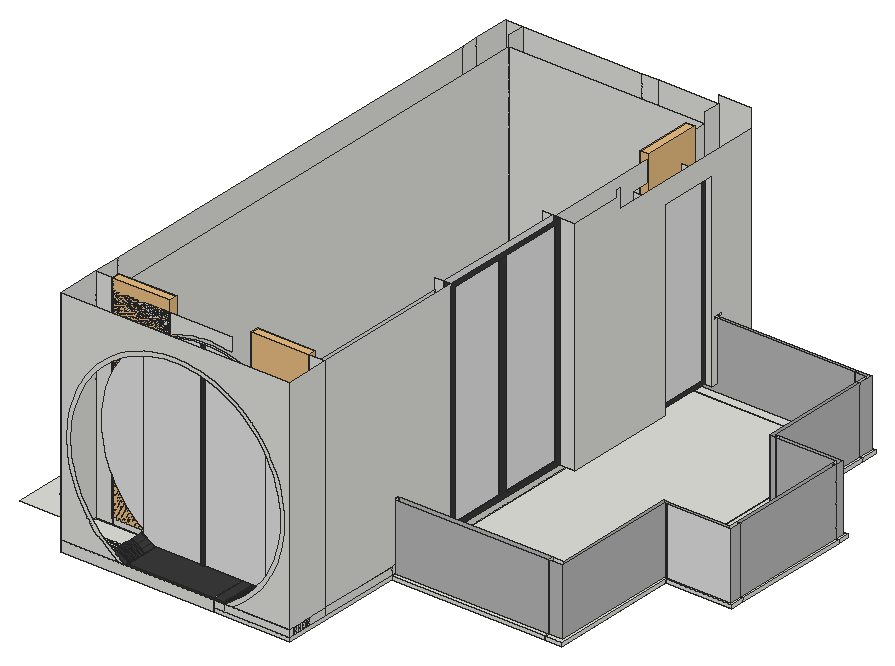
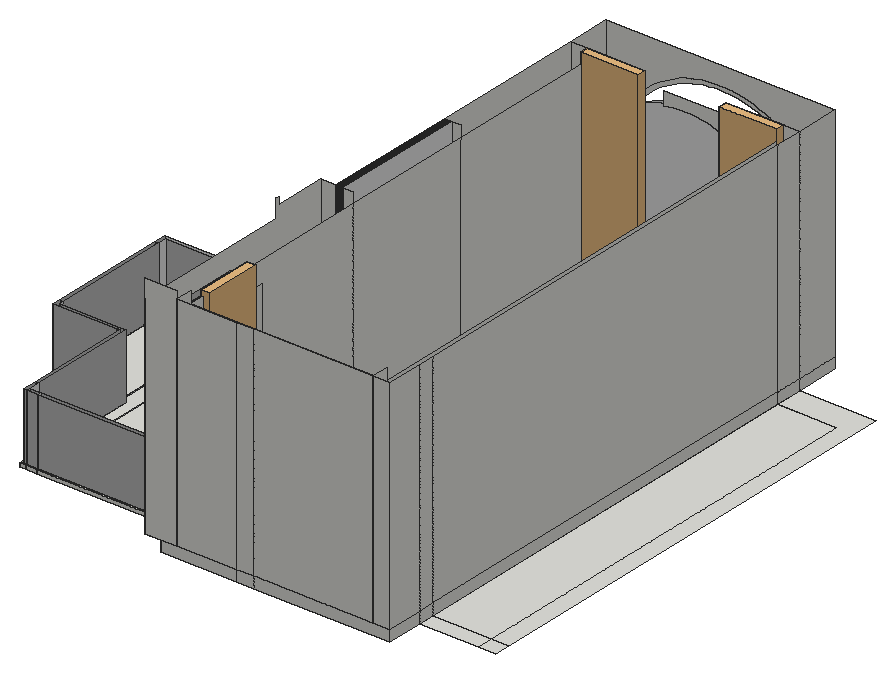
# SketchUp Ruby script. Lengths in inches.
U = 1.inch
M = Sketchup.active_model
def pt(a) = Geom::Point3d.new(a.map { |v| v * U })
def face(e, loops, mat)
  f = e.add_face(loops[0].map { |a| pt(a) })
  loops[1..].each { |l| e.add_face(l.map { |a| pt(a) }).erase! }
  f.material = f.back_material = mat if mat
  f
end
# faces: each face lists its corners as indices into pts; further lists are holes
def faces(e, pts, list, mat = nil) = list.each { |f| face(e, (f[0].is_a?(Array) ? f : [f]).map { |l| l.map { |i| pts[i] } }, mat) }
# xy, xz, yz: faces in a plane at the given z, y or x. An outline is a flat list of corners, or four numbers for a rectangle; further outlines are holes
def ring(l) = l.size == 4 ? [[l[0], l[1]], [l[2], l[1]], [l[2], l[3]], [l[0], l[3]]] : l.each_slice(2).to_a
def flat(e, list, mat, &to3) = list.each { |f| face(e, (f[0].is_a?(Array) ? f : [f]).map { |l| ring(l).map { |u, v| to3.(u, v) } }, mat) }
def xy(e, z, list, mat = nil) = flat(e, list, mat) { |x, y| [x, y, z] }
def xz(e, y, list, mat = nil) = flat(e, list, mat) { |x, z| [x, y, z] }
def yz(e, x, list, mat = nil) = flat(e, list, mat) { |y, z| [x, y, z] }
def lines(e, pts, list) = list.each { |a, b| e.add_line(pt(pts[a]), pt(pts[b])) }
# prism: a flat outline (further loops are holes) pulled along v
def prism(e, loops, v, mat = nil)
  f = face(e, loops, mat); d = Geom::Vector3d.new(v.map { |x| x * U })
  f.pushpull(f.normal.samedirection?(d) ? d.length : -d.length)
end
def box(e, o, s, mat = nil) = prism(e, [[o, [o[0] + s[0], o[1], o[2]], [o[0] + s[0], o[1] + s[1], o[2]], [o[0], o[1] + s[1], o[2]]]], [0, 0, s[2]], mat)
def at(x, y, z, deg = 0) = Geom::Transformation.translation(pt([x, y, z])) * Geom::Transformation.rotation(ORIGIN, Z_AXIS, deg.degrees)
def axes(o, x, y, z) = Geom::Transformation.new([*x, 0, *y, 0, *z, 0, *pt(o).to_a, 1])
def part(name) = M.definitions.add(name)
# library, detail: a bought-in or finely detailed component or shape, given as its bounding box
def library(name, o, s) = part(name).tap { |d| box(d.entities, o, s) }
def detail(e, o, s) = box(e.add_group.entities, o, s)
def put(e, d, t, mat = nil) = e.add_instance(d, t).tap { |i| i.material = mat if mat }
def group(e, t, mat = nil) = e.add_group.tap { |g| g.transformation = t; g.material = mat if mat }.entities
root = M.entities
M.materials.add("[Color M07]").color = [58, 58, 58]
M.materials.add("[Mirror 01]").color = [185, 185, 185]
M.materials.add("[Mirror 02]").color = [229, 229, 229]
c1 = library("Curtains 004",[-15.59,-2.26,0],[31.18,4.52,116.91])
xy(root,120,[[115,13.45,115,52.07,41.2,52.07,41.2,37.13,124,37.13,124,13.45],[41.2,13.45,115,37.13],[[115,13.45,115,37.13,41.2,37.13,41.2,295.13,115,295.13,115,315.2,124,315.2,124,295.13,165.63,295.13,165.63,106.13,126,106.13,126,82.13,165.63,82.13,165.63,13.45],[115,286.13,124,295.13]],[124,13.45,165.63,13.45,165.63,295.13,124,295.13,124,286.13,249,286.13,249,106.13,124,106.13],[0,37.13,41.2,37.13,41.2,52.07,9,52.07,9,286.13,0,286.13],
  [41.2,37.13,41.2,295.13,115,295.13,115,286.13,9,286.13,9,52.07,115,52.07,115,37.13],[126,82.13,165.63,94.13],[165.63,82.13,249,94.13],[249,82.13,258,286.13],[126,94.13,165.63,95.7],
  [165.63,94.13,249,95.7],[126,95.7,165.63,106.13],[165.63,95.7,249,106.13],[258,152.76,294,160.01],[258,160.01,294,224.82],
  [258,224.82,294,230.88],[0,286.13,9,295.13],[9,286.13,41.2,295.13],[41.2,286.13,115,295.13],[115,286.13,124,295.13],
  [124,286.13,165.63,295.13],[165.63,286.13,249,295.13],[249,286.13,255,295.13],[255,286.13,258,295.13],[115,295.13,124,315.2],
  [124,295.13,165.63,315.2]])
xy(root,122,[[124,13.45,165.63,106.13],[165.63,82.13,249,84.55],[249,82.13,258,82.13,258,153.49,256.57,153.49,256.57,84.55,249,84.55],[165.63,84.55,249,87.25],[249,84.55,249,87.25,255,87.25,255,155.13,258,155.13,258,153.49,256.57,153.49,256.57,84.55],
  [165.63,87.25,249,94.13],[249,87.25,249,286.13,255,286.13,255,227.13,258,227.13,258,155.13,255,155.13,255,87.25],[165.63,94.13,249,94.2],[165.63,94.2,238.38,95.7],[238.38,94.2,249,95.7],
  [165.63,95.7,238.38,106.13],[238.38,95.7,249,106.13],[165.63,106.13,165.63,295.13,124,295.13,124,286.13,249,286.13,249,106.13],[258,152.76,294,152.76,294,160.01,292.7,160.01,292.7,153.49,258,153.49],[258,153.49,258,155.13,290.75,155.13,290.75,160.01,292.7,160.01,292.7,153.49],
  [258,155.13,290.75,160.01],[258,160.01,290.75,224.82],[290.75,160.01,292.7,224.82],[292.7,160.01,294,224.82],[258,224.82,290.75,227.13],
  [290.75,224.82,290.75,227.13,258,227.13,258,229.11,292.7,229.11,292.7,224.82],[292.7,224.82,294,224.82,294,230.88,258,230.88,258,229.11,292.7,229.11],[255,227.13,255,286.13,256.57,286.13,256.57,229.11,258,229.11,258,227.13],[256.57,229.11,258,286.13],[165.63,286.13,249,292.13],
  [249,286.13,255,292.13],[255,286.13,256.57,293.99],[256.57,286.13,258,286.13,258,295.13,255,295.13,255,293.99,256.57,293.99],[165.63,292.13,249,293.99],[249,292.13,255,293.99],
  [165.63,293.99,249,295.13],[249,293.99,255,295.13]])
xy(root,122.625,[[165.63,87.25,249,94.13],[249,87.25,255,87.25,255,155.13,258,155.13,258,227.13,255,227.13,255,286.13,249,286.13],[165.63,94.2,238.38,95.7],[238.38,94.2,249,95.7],[165.63,95.7,238.38,106.13],
  [238.38,95.7,249,106.13],[165.63,106.13,249,106.13,249,286.13,124,286.13,124,295.13,165.63,295.13],[258,160.01,290.75,224.82]])
xy(root,126,[[41.2,13.45,77.2,14.95],[77.2,13.45,77.2,33.16,101.89,33.16,101.89,32.53,103.41,32.53,103.41,33.16,124,33.16,124,13.45],[124,13.45,129.63,33.16],[129.63,13.45,165.63,14.95],[41.2,14.95,77.2,15.8],
  [129.63,14.95,165.63,15.8],[41.2,15.8,77.2,16.65],[129.63,15.8,165.63,16.65],[41.2,16.65,77.2,17.5],[129.63,16.65,165.63,17.5],
  [41.2,17.5,77.2,18.35],[129.63,17.5,165.63,18.35],[41.2,18.35,77.2,19.21],[129.63,18.35,165.63,19.21],[41.2,19.21,77.2,19.95],
  [129.63,19.21,165.63,19.95],[41.2,19.95,77.2,21.02],[129.63,19.95,165.63,21.02],[41.2,21.02,77.2,22.08],[129.63,21.02,165.63,22.08],
  [41.2,22.08,77.2,23.14],[129.63,22.08,165.63,23.14],[41.2,23.14,77.2,24.2],[129.63,23.14,165.63,24.2],[41.2,24.2,77.2,25.27],
  [129.63,24.2,165.63,25.27],[41.2,25.27,77.2,26.33],[129.63,25.27,165.63,26.33],[41.2,26.33,77.2,37.13],[129.63,26.33,165.63,37.13],
  [101.89,32.53,103.41,33.16],[77.2,33.16,124,34.78],[124,33.16,129.63,34.78],[77.2,34.78,124,37.13],[124,34.78,129.63,37.13],
  [41.2,37.13,124,37.13,124,106.13,156.63,106.13,156.63,286.13,124,286.13,124,295.13,156.63,295.13,156.63,306.2,50.2,306.2,50.2,37.45,41.2,37.45],[124,37.13,156.63,106.13],[156.63,37.13,165.63,106.13],[41.2,37.45,50.2,315.2],[156.63,106.13,165.63,122.64],
  [156.63,122.64,161.76,196.13],[156.63,196.13,165.63,256.99],[165.63,196.13,174.13,256.99],[156.63,256.99,165.63,286.13],[124,286.13,156.63,295.13],
  [156.63,286.13,165.63,288.98],[156.63,288.98,165.63,295.13],[165.63,288.98,174.13,292.13],[165.63,293.99,174.13,295.13],[156.63,295.13,165.63,315.2],
  [165.63,295.13,174.13,315.2],[50.2,306.2,156.63,315.2]])
xy(root,126,[[161.76,122.64,165.63,196.13],[168.07,256.99,169.88,286.13],[168.07,286.13,169.88,288.98]],"[Color M07]")
xy(root,126.625,[[77.2,13.45,124,13.45,124,33.16,103.41,33.16,103.41,32.53,101.89,32.53,101.89,33.16,77.2,33.16],[124,13.45,129.63,33.16]],"[Color M07]")
xy(root,127.86,[[169.38,258.85,169.88,286.13],[169.38,286.13,169.88,287.12]],"[Color M07]")
xy(root,128.57,[[164.38,125.2,165.63,155.73],[164.38,159.39,165.63,193.57]],"[Color M07]")
xz(root,13.45,[[41.2,120,124,126],[124,120,165.63,122],[124,122,129.63,126],[129.63,122,165.63,126],[41.2,126,72.37,126,69.11,128.28,68.1,128.99,65.61,130.93,63.22,133.01,60.95,135.22,58.8,137.54,56.78,139.97,54.89,142.51,53.13,145.14,51.52,147.86,50.06,150.67,48.75,153.55,47.59,156.49,46.59,159.49,45.75,162.54,45.08,165.64,44.57,168.76,44.23,171.9,44.0625,175.0625,44.06,178.23,44.22,181.39,44.55,184.53,45.05,187.66,45.72,190.75,46.55,193.8,47.54,196.81,48.6875,199.75,49.99,202.64,51.45,205.45,53.05,208.17,54.8,210.81,56.6875,213.35,58.7,215.79,60.85,218.11,63.11,220.32,65.49,222.41,67.98,224.36,70.57,226.18,73.25,227.86,76.02,229.4,78.86,230.78,81.78,232.01,84.75,233.09,87.78,234,90.85,234.75,93.96,235.34,97.1,235.76,100.25,236.01,103.41,236.1,106.58,236.01,109.73,235.76,112.87,235.34,115.98,234.75,119.05,234,122.08,233.09,125.05,232.01,127.97,230.78,130.8125,229.4,133.58,227.86,136.26,226.18,138.85,224.36,141.34,222.41,143.72,220.32,145.98,218.11,148.125,215.79,150.14,213.35,152.03,210.81,153.78,208.17,155.38,205.45,156.84,202.64,158.14,199.75,159.29,196.81,160.28,193.8,161.11,190.75,161.78,187.66,162.28,184.53,162.61,181.39,162.77,178.23,162.77,175.0625,162.6,171.9,162.26,168.76,161.75,165.64,161.08,162.54,160.24,159.49,159.24,156.49,158.08,153.55,156.77,150.67,155.31,147.86,153.7,145.14,151.94,142.51,150.05,139.97,148.03,137.54,145.88,135.22,143.61,133.01,141.22,130.93,138.73,128.99,137.72,128.28,134.46,126,165.63,126,165.63,246,41.2,246],
  [72.37,126,77.2,126,74.53,127.47,71.95,129.08,69.46,130.82,67.06,132.69,64.77,134.69,62.58,136.8125,60.52,139.04,58.57,141.38,56.75,143.82,55.07,146.35,53.52,148.97,52.11,151.67,50.85,154.4375,49.74,157.27,48.78,160.15,47.97,163.09,47.32,166.0625,46.84,169.0625,46.51,172.09,46.34,175.125,46.34,178.17,46.5,181.21,46.82,184.23,47.3,187.24,47.9375,190.21,48.73,193.15,49.6875,196.03,50.79,198.87,52.05,201.64,53.45,204.34,54.99,206.96,56.67,209.5,58.48,211.94,60.42,214.29,62.48,216.52,64.66,218.65,66.95,220.65,69.34,222.53,71.83,224.28,74.41,225.9,77.07,227.37,79.81,228.7,82.61,229.89,85.47,230.92,88.38,231.8,91.34,232.52,94.33,233.08,97.34,233.49,100.375,233.73,103.41,233.8125,106.46,233.73,109.49,233.49,112.5,233.08,115.49,232.52,118.45,231.8,121.36,230.92,124.22,229.89,127.02,228.7,129.76,227.37,132.42,225.9,135,224.28,137.49,222.53,139.88,220.65,142.17,218.65,144.35,216.52,146.41,214.29,148.35,211.94,150.16,209.5,151.84,206.96,153.38,204.34,154.78,201.64,156.04,198.87,157.14,196.03,158.09,193.15,158.89,190.21,159.53,187.24,160.01,184.23,160.33,181.21,160.49,178.17,160.49,175.125,160.32,172.09,159.99,169.0625,159.51,166.0625,158.86,163.09,158.05,160.15,157.09,157.27,155.98,154.4375,154.72,151.67,153.3125,148.97,151.76,146.35,150.08,143.82,148.26,141.38,146.3125,139.04,144.25,136.8125,142.0625,134.69,139.77,132.69,137.375,130.82,134.88,129.08,132.3,127.47,129.63,126,134.46,126,137.72,128.28,138.73,128.99,141.22,130.93,143.61,133.01,145.88,135.22,148.03,137.54,150.05,139.97,151.94,142.51,153.7,145.14,155.31,147.86,156.77,150.67,158.08,153.55,159.24,156.49,160.24,159.49,161.08,162.54,161.75,165.64,162.26,168.76,162.6,171.9,162.77,175.0625,162.77,178.23,162.61,181.39,162.28,184.53,161.78,187.66,161.11,190.75,160.28,193.8,159.29,196.81,158.14,199.75,156.84,202.64,155.38,205.45,153.78,208.17,152.03,210.81,150.14,213.35,148.125,215.79,145.98,218.11,143.72,220.32,141.34,222.41,138.85,224.36,136.26,226.18,133.58,227.86,130.8125,229.4,127.97,230.78,125.05,232.01,122.08,233.09,119.05,234,115.98,234.75,112.87,235.34,109.73,235.76,106.58,236.01,103.41,236.1,100.25,236.01,97.1,235.76,93.96,235.34,90.85,234.75,87.78,234,84.75,233.09,81.78,232.01,78.86,230.78,76.02,229.4,73.25,227.86,70.57,226.18,67.98,224.36,65.49,222.41,63.11,220.32,60.85,218.11,58.7,215.79,56.6875,213.35,54.8,210.81,53.05,208.17,51.45,205.45,49.99,202.64,48.6875,199.75,47.54,196.81,46.55,193.8,45.72,190.75,45.05,187.66,44.55,184.53,44.22,181.39,44.06,178.23,44.0625,175.0625,44.23,171.9,44.57,168.76,45.08,165.64,45.75,162.54,46.59,159.49,47.59,156.49,48.75,153.55,50.06,150.67,51.52,147.86,53.13,145.14,54.89,142.51,56.78,139.97,58.8,137.54,60.95,135.22,63.22,133.01,65.61,130.93,68.1,128.99,69.11,128.28]])
xz(root,13.45,[[77.2,126,124,126.625],[124,126,129.63,126.625]],"[Color M07]")
xz(root,32.53,[[101.89,126,103.41,126.625]])
xz(root,32.53,[[101.89,126.625,103.41,126.625,103.41,233.8125,101.89,233.77]],"[Color M07]")
xz(root,33.16,[[77.2,126,101.89,126.625],[101.89,126,101.89,233.77,103.41,233.8125,103.41,126],[103.41,126,124,126.625],[124,126,129.63,126.625]])
xz(root,33.16,[[77.2,126,77.2,126.625,101.89,126.625,101.89,233.77,100.375,233.73,97.34,233.49,94.33,233.08,91.34,232.52,88.38,231.8,85.47,230.92,82.61,229.89,79.81,228.7,77.07,227.37,74.41,225.9,71.83,224.28,70.64,223.45,70.64,129.99,71.95,129.08,74.53,127.47],[129.63,126,132.3,127.47,134.88,129.08,136.24,130.03,136.24,223.41,135,224.28,132.42,225.9,129.76,227.37,127.02,228.7,124.22,229.89,121.36,230.92,118.45,231.8,115.49,232.52,112.5,233.08,109.49,233.49,106.46,233.73,103.41,233.8125,103.41,126.625,129.63,126.625]],"[Mirror 02]")
xz(root,34.78,[[77.2,126,74.53,127.47,71.95,129.08,69.46,130.82,67.06,132.69,64.77,134.69,62.58,136.8125,60.52,139.04,58.57,141.38,56.75,143.82,55.07,146.35,53.52,148.97,52.11,151.67,50.85,154.4375,49.74,157.27,48.78,160.15,47.97,163.09,47.32,166.0625,46.84,169.0625,46.51,172.09,46.34,175.125,46.34,178.17,46.5,181.21,46.82,184.23,47.3,187.24,47.9375,190.21,48.73,193.15,49.6875,196.03,50.79,198.87,52.05,201.64,53.45,204.34,54.99,206.96,56.67,209.5,58.48,211.94,60.42,214.29,62.48,216.52,64.66,218.65,66.95,220.65,69.34,222.53,71.83,224.28,74.41,225.9,77.07,227.37,79.81,228.7,82.61,229.89,85.47,230.92,88.38,231.8,91.34,232.52,94.33,233.08,97.34,233.49,100.375,233.73,103.41,233.8125,106.46,233.73,109.49,233.49,112.5,233.08,115.49,232.52,118.45,231.8,121.36,230.92,124.22,229.89,127.02,228.7,129.76,227.37,132.42,225.9,135,224.28,137.49,222.53,139.88,220.65,142.17,218.65,144.35,216.52,146.41,214.29,148.35,211.94,150.16,209.5,151.84,206.96,153.38,204.34,154.78,201.64,156.04,198.87,157.14,196.03,158.09,193.15,158.89,190.21,159.53,187.24,160.01,184.23,160.33,181.21,160.49,178.17,160.49,175.125,160.32,172.09,159.99,169.0625,159.51,166.0625,158.86,163.09,158.05,160.15,157.09,157.27,155.98,154.4375,154.72,151.67,153.3125,148.97,151.76,146.35,150.08,143.82,148.26,141.38,146.3125,139.04,144.25,136.8125,142.0625,134.69,139.77,132.69,137.375,130.82,134.88,129.08,132.3,127.47,129.63,126]],"[Mirror 02]")
xz(root,37.13,[[41.2,120,115,126],[41.2,126,41.2,246,50.2,246,50.2,240,115,240,115,232.61,112.5,233.08,109.49,233.49,106.46,233.73,103.41,233.8125,100.375,233.73,97.34,233.49,94.33,233.08,91.34,232.52,88.38,231.8,85.47,230.92,82.61,229.89,79.81,228.7,77.07,227.37,74.41,225.9,71.83,224.28,69.34,222.53,66.95,220.65,64.66,218.65,62.48,216.52,60.42,214.29,58.48,211.94,56.67,209.5,54.99,206.96,53.45,204.34,52.05,201.64,50.79,198.87,49.6875,196.03,48.73,193.15,47.9375,190.21,47.3,187.24,46.82,184.23,46.5,181.21,46.34,178.17,46.34,175.125,46.51,172.09,46.84,169.0625,47.32,166.0625,47.97,163.09,48.78,160.15,49.74,157.27,50.85,154.4375,52.11,151.67,53.52,148.97,55.07,146.35,56.75,143.82,58.57,141.38,60.52,139.04,62.58,136.8125,64.77,134.69,67.06,132.69,69.46,130.82,71.95,129.08,74.53,127.47,77.2,126],[129.63,126,132.3,127.47,134.88,129.08,137.375,130.82,139.77,132.69,142.0625,134.69,144.25,136.8125,146.3125,139.04,148.26,141.38,150.08,143.82,151.76,146.35,153.3125,148.97,154.72,151.67,155.98,154.4375,156.63,156.1,156.63,126],[156.63,126,156.63,156.1,157.09,157.27,158.05,160.15,158.86,163.09,159.51,166.0625,159.99,169.0625,160.32,172.09,160.49,175.125,160.49,178.17,160.33,181.21,160.01,184.23,159.53,187.24,158.89,190.21,158.09,193.15,157.14,196.03,156.63,197.34,156.63,246,165.63,246,165.63,126]])
xz(root,37.45,[[41.2,126,50.2,246]])
xz(root,82.13,[[165.63,120,249,122],[249,120,258,122]])
xz(root,84.55,[[165.63,122,249,158],[249,122,256.57,158]],"[Mirror 01]")
xz(root,87.25,[[165.63,122,249,122.625],[249,122,255,122.625],[249,122.625,255,158]])
xz(root,87.25,[[165.63,122.625,249,158]],"[Mirror 01]")
xz(root,94.13,[[165.63,120,249,122],[165.63,122,249,122.625]])
xz(root,94.2,[[165.63,122,238.38,122.625],[238.38,122,249,122.625]])
xz(root,95.7,[[165.63,120,249,122],[165.63,122,238.38,122.625],[238.38,122,249,122.625]])
xz(root,106.13,[[124,120,126,122],[126,120,165.63,122],[165.63,120,249,122],[124,122,126,126],[126,122,156.63,126],
  [156.63,122,165.63,126],[165.63,122,238.38,122.625],[238.38,122,249,122.625]])
xz(root,122.64,[[156.63,126,161.76,246]])
xz(root,122.64,[[161.76,126,165.63,246]],"[Color M07]")
xz(root,125.2,[[164.38,128.57,165.63,243.43]],"[Color M07]")
xz(root,152.76,[[258,120,294,122]])
xz(root,153.49,[[256.57,122,258,158]])
xz(root,153.49,[[258,122,292.7,158]],"[Mirror 02]")
xz(root,155.13,[[255,122,258,122.625]])
xz(root,155.13,[[258,122,290.75,158],[255,122.625,258,158]],"[Mirror 01]")
xz(root,155.73,[[164.38,128.57,165.63,243.43]],"[Color M07]")
xz(root,159.39,[[164.38,128.57,165.63,243.43]],"[Color M07]")
xz(root,160.01,[[258,120,294,122],[258,122,290.75,122.625],[290.75,122,292.7,158]])
xz(root,193.57,[[164.38,128.57,165.63,243.43]])
xz(root,196.13,[[156.63,126,161.76,246],[165.63,126,174.13,246]])
xz(root,196.13,[[161.76,126,165.63,246]],"[Color M07]")
xz(root,224.82,[[258,120,294,122],[258,122,290.75,122.625],[290.75,122,292.7,158]])
xz(root,227.13,[[255,122,258,122.625]])
xz(root,227.13,[[258,122,290.75,158],[255,122.625,258,158]],"[Mirror 01]")
xz(root,229.11,[[256.57,122,258,158],[258,122,292.7,158]],"[Mirror 01]")
xz(root,230.88,[[258,120,294,122]])
xz(root,256.99,[[156.63,126,168.07,228.5625],[169.88,126,174.13,228.5625]])
xz(root,256.99,[[168.07,126,169.88,228.5625]],"[Color M07]")
xz(root,258.85,[[169.38,127.86,169.88,226.7]],"[Color M07]")
xz(root,286.13,[[124,120,165.63,122],[165.63,120,249,122],[249,120,255,122],[255,120,258,122],[124,122,156.63,122.625],
  [156.63,122,165.63,122.625],[165.63,122,249,122.625],[249,122,255,122.625],[255,122,256.57,158],[124,122.625,156.63,126],
  [156.63,122.625,165.63,126]])
xz(root,287.12,[[169.38,127.86,169.88,226.7]],"[Color M07]")
xz(root,288.98,[[156.63,126,168.07,228.5625],[169.88,126,174.13,228.5625]])
xz(root,288.98,[[168.07,126,169.88,228.5625]],"[Color M07]")
xz(root,292.13,[[165.63,126,174.13,158]])
xz(root,292.13,[[165.63,122,249,122,249,158,174.13,158,174.13,126,165.63,126],[249,122,255,158]],"[Mirror 01]")
xz(root,293.99,[[165.63,126,174.13,158]])
xz(root,293.99,[[165.63,122,165.63,126,174.13,126,174.13,158,249,158,249,122],[249,122,255,158],[255,122,256.57,158]],"[Mirror 01]")
xz(root,295.13,[[124,120,165.63,122],[165.63,120,249,122],[249,120,255,122],[255,120,258,122],[124,122,156.63,122.625],
  [156.63,122,165.63,122.625],[124,122.625,156.63,126],[156.63,122.625,165.63,126]])
xz(root,306.2,[[50.2,126,156.63,240]])
xz(root,315.2,[[41.2,120,115,126],[115,120,124,126],[124,120,165.63,126],[41.2,126,50.2,246],[50.2,126,115,246],
  [115,126,124,246],[124,126,156.63,246],[156.63,126,174.13,250.0625]])
yz(root,41.2,[[13.45,120,37.13,126],[37.13,120,52.07,126],[52.07,120,286.13,126],[286.13,120,295.13,126],[295.13,120,315.2,126],
  [13.45,126,37.13,246],[37.45,126,52.07,246],[52.07,126,286.13,246],[286.13,126,295.13,246],[295.13,126,315.2,246]])
yz(root,50.2,[[37.45,126,306.2,240],[306.2,126,315.2,246]])
yz(root,77.2,[[13.45,126,14.95,126.625],[14.95,126,15.8,126.625],[15.8,126,16.65,126.625],[16.65,126,17.5,126.625],[17.5,126,18.35,126.625],
  [18.35,126,19.21,126.625],[19.21,126,19.95,126.625],[19.95,126,21.02,126.625],[21.02,126,22.08,126.625],[22.08,126,23.14,126.625],
  [23.14,126,24.2,126.625],[24.2,126,25.27,126.625],[25.27,126,26.33,126.625],[26.33,126,33.16,126.625]],"[Color M07]")
yz(root,101.89,[[32.53,126,33.16,126.625]])
yz(root,101.89,[[32.53,126.625,33.16,233.77]],"[Color M07]")
yz(root,103.41,[[32.53,126,33.16,126.625]])
yz(root,103.41,[[32.53,126.625,33.16,233.8125]],"[Color M07]")
yz(root,124,[[13.45,120,37.13,122],[37.13,120,46.13,122],[46.13,120,106.13,122],[286.13,120,295.13,122],[13.45,122,33.16,126],
  [33.16,122,34.78,126],[34.78,122,37.13,126],[37.13,122,46.13,126],[46.13,122,106.13,126],[286.13,122,295.13,122.625],
  [286.13,122.625,295.13,126],[13.45,126,33.16,126.625]])
yz(root,129.63,[[13.45,126,14.95,126.625],[14.95,126,15.8,126.625],[15.8,126,16.65,126.625],[16.65,126,17.5,126.625],[17.5,126,18.35,126.625],
  [18.35,126,19.21,126.625],[19.21,126,19.95,126.625],[19.95,126,21.02,126.625],[21.02,126,22.08,126.625],[22.08,126,23.14,126.625],
  [23.14,126,24.2,126.625],[24.2,126,25.27,126.625],[25.27,126,26.33,126.625],[26.33,126,33.16,126.625]],"[Color M07]")
yz(root,156.63,[[37.13,126,122.64,240],[122.64,126,196.13,240],[196.13,126,196.13,240,306.2,240,306.2,126,288.98,126,288.98,228.5625,256.99,228.5625,256.99,126],[306.2,126,315.2,246]])
yz(root,161.76,[[122.64,126,196.13,246]],"[Mirror 02]")
yz(root,164.38,[[125.2,128.57,155.73,243.43],[159.39,128.57,193.57,243.43]],"[Mirror 02]")
yz(root,165.63,[[13.45,120,82.13,122],[82.13,120,87.25,122],[87.25,120,94.13,122],[94.13,120,95.7,122],[95.7,120,106.13,122],
  [106.13,120,286.13,122],[286.13,120,295.13,122],[295.13,120,315.2,126],[13.45,122,14.95,126],[14.95,122,15.8,126],
  [15.8,122,16.65,126],[16.65,122,17.5,126],[17.5,122,18.35,126],[18.35,122,19.21,126],[19.21,122,19.95,126],
  [19.95,122,21.02,126],[21.02,122,22.08,126],[22.08,122,23.14,126],[23.14,122,24.2,126],[24.2,122,25.27,126],
  [25.27,122,26.33,126],[26.33,122,37.13,126],[37.13,122,82.13,126],[82.13,122,84.55,126],[84.55,122,87.25,126],
  [87.25,122,94.13,122.625],[94.13,122,94.2,122,94.2,122.625,95.7,122.625,95.7,126,94.13,126],[94.2,122,95.7,122.625],[95.7,122,106.13,122.625],[106.13,122,286.13,122.625],
  [286.13,122,292.13,122.625],[292.13,122,293.99,122.625],[293.99,122,295.13,122.625],[87.25,122.625,94.13,126],[95.7,122.625,106.13,126],
  [106.13,122.625,286.13,126],[286.13,122.625,292.13,126],[292.13,122.625,293.99,126],[293.99,122.625,295.13,126],[13.45,126,37.13,246],
  [37.13,126,84.55,126,84.55,158.5625,87.25,158.5625,87.25,126,122.64,126,122.64,246,37.13,246],[84.55,126,87.25,158],[292.13,126,293.99,158]])
yz(root,165.63,[[[122.64,126,196.13,246],[125.2,128.57,193.57,243.43]],[155.73,128.57,159.39,243.43]],"[Color M07]")
yz(root,168.07,[[256.99,126,288.98,228.5625]],"[Mirror 02]")
yz(root,169.38,[[258.85,127.86,287.12,226.7]],"[Mirror 02]")
yz(root,169.88,[[[256.99,126,288.98,228.5625],[258.85,127.86,287.12,226.7]]],"[Color M07]")
yz(root,174.13,[[196.13,126,256.99,126,256.99,228.5625,288.98,228.5625,288.98,126,292.13,126,292.13,158,289.77,158,289.77,159.75,295.59,159.75,295.59,158,293.99,158,293.99,126,315.2,126,315.2,239.89,226.42,239.89,226.42,250.0625,224.6,250.0625,224.6,246,196.13,246]])
yz(root,238.38,[[94.2,122,95.7,122.625],[95.7,122,106.13,122.625]])
yz(root,249,[[82.13,120,87.25,122],[87.25,120,94.13,122],[94.13,120,95.7,122],[95.7,120,106.13,122],[106.13,120,286.13,122],
  [286.13,120,295.13,122],[84.55,122,87.25,158],[87.25,122,94.13,122.625],[94.13,122,94.2,122.625],[94.2,122,95.7,122.625],
  [95.7,122,106.13,122.625],[106.13,122,286.13,122.625],[292.13,122,293.99,158]])
yz(root,255,[[286.13,120,295.13,122],[87.25,122,155.13,122.625],[227.13,122,286.13,122.625],[292.13,122,293.99,158]])
yz(root,255,[[87.25,122.625,155.13,158],[227.13,122.625,286.13,158]],"[Mirror 01]")
yz(root,255,[[286.13,122,292.13,158]],"[Mirror 02]")
yz(root,256.57,[[84.55,122,153.49,158],[229.11,122,286.13,158],[286.13,122,293.99,158]],"[Mirror 01]")
yz(root,258,[[82.13,120,152.76,122],[152.76,120,160.01,122],[160.01,120,224.82,122],[224.82,120,230.88,122],[230.88,120,286.13,122],
  [286.13,120,295.13,122],[153.49,122,155.13,158],[155.13,122,160.01,122.625],[160.01,122,224.82,122.625],[224.82,122,227.13,122.625],
  [227.13,122,229.11,158]])
yz(root,290.75,[[160.01,122,224.82,122.625]])
yz(root,290.75,[[160.01,122.625,224.82,158]],"[Mirror 01]")
yz(root,290.75,[[155.13,122,160.01,158],[224.82,122,227.13,158]],"[Mirror 02]")
yz(root,292.7,[[153.49,122,160.01,158],[160.01,122,224.82,158],[224.82,122,229.11,158]],"[Mirror 01]")
yz(root,294,[[152.76,120,160.01,122],[160.01,120,224.82,122],[224.82,120,230.88,122]])
p = [[77.2,13.45,126],[77.2,14.95,126],[74.53,14.95,127.47],[74.53,13.45,127.47],[132.3,13.45,127.47],[132.3,14.95,127.47],
  [129.63,14.95,126],[129.63,13.45,126],[77.2,15.8,126],[74.53,15.8,127.47],[132.3,15.8,127.47],[129.63,15.8,126],
  [77.2,16.65,126],[74.53,16.65,127.47],[132.3,16.65,127.47],[129.63,16.65,126],[77.2,17.5,126],[74.53,17.5,127.47],
  [132.3,17.5,127.47],[129.63,17.5,126],[77.2,18.35,126],[74.53,18.35,127.47],[132.3,18.35,127.47],[129.63,18.35,126],
  [77.2,19.21,126],[74.53,19.21,127.47],[132.3,19.21,127.47],[129.63,19.21,126],[77.2,19.95,126],[74.53,19.95,127.47],
  [132.3,19.95,127.47],[129.63,19.95,126],[77.2,21.02,126],[74.53,21.02,127.47],[132.3,21.02,127.47],[129.63,21.02,126],
  [77.2,22.08,126],[74.53,22.08,127.47],[132.3,22.08,127.47],[129.63,22.08,126],[77.2,23.14,126],[74.53,23.14,127.47],
  [132.3,23.14,127.47],[129.63,23.14,126],[77.2,24.2,126],[74.53,24.2,127.47],[132.3,24.2,127.47],[129.63,24.2,126],
  [77.2,25.27,126],[74.53,25.27,127.47],[132.3,25.27,127.47],[129.63,25.27,126],[77.2,26.33,126],[74.53,26.33,127.47],
  [132.3,26.33,127.47],[129.63,26.33,126],[77.2,33.16,126],[74.53,33.16,127.47],[132.3,33.16,127.47],[129.63,33.16,126],
  [74.53,34.78,127.47],[77.2,34.78,126],[129.63,34.78,126],[132.3,34.78,127.47],[74.53,37.13,127.47],[77.2,37.13,126],
  [129.63,37.13,126],[132.3,37.13,127.47],[71.95,14.95,129.08],[71.95,13.45,129.08],[134.88,13.45,129.08],[134.88,14.95,129.08],
  [71.95,15.8,129.08],[134.88,15.8,129.08],[71.95,16.65,129.08],[134.88,16.65,129.08],[71.95,17.5,129.08],[134.88,17.5,129.08],
  [71.95,18.35,129.08],[134.88,18.35,129.08],[71.95,19.21,129.08],[134.88,19.21,129.08],[71.95,19.95,129.08],[134.88,19.95,129.08],
  [71.95,21.02,129.08],[134.88,21.02,129.08],[71.95,22.08,129.08],[134.88,22.08,129.08],[71.95,23.14,129.08],[134.88,23.14,129.08],
  [71.95,24.2,129.08],[134.88,24.2,129.08],[71.95,25.27,129.08],[134.88,25.27,129.08],[71.95,26.33,129.08],[134.88,26.33,129.08],
  [71.95,33.16,129.08],[134.88,33.16,129.08],[71.95,34.78,129.08],[134.88,34.78,129.08],[71.95,37.13,129.08],[134.88,37.13,129.08],
  [69.46,14.95,130.82],[69.46,13.45,130.82],[137.375,13.45,130.82],[137.375,14.95,130.82],[69.46,15.8,130.82],[137.375,15.8,130.82],
  [69.46,16.65,130.82],[137.375,16.65,130.82],[69.46,17.5,130.82],[137.375,17.5,130.82],[69.46,18.35,130.82],[137.375,18.35,130.82],
  [69.46,19.21,130.82],[137.375,19.21,130.82],[69.46,19.95,130.82],[137.375,19.95,130.82],[69.46,21.02,130.82],[137.375,21.02,130.82],
  [69.46,22.08,130.82],[137.375,22.08,130.82],[69.46,23.14,130.82],[137.375,23.14,130.82],[69.46,24.2,130.82],[137.375,24.2,130.82],
  [69.46,25.27,130.82],[137.375,25.27,130.82],[69.46,26.33,130.82],[137.375,26.33,130.82],[70.64,33.16,129.99],[70.64,32.53,129.99],
  [69.46,32.53,130.82],[136.24,32.53,130.03],[136.24,33.16,130.03],[137.375,32.53,130.82],[69.46,34.78,130.82],[69.46,33.16,130.82],
  [137.375,34.78,130.82],[137.375,33.16,130.82],[69.46,37.13,130.82],[137.375,37.13,130.82],[126,82.13,120],[126,82.13,126],
  [126,95.7,120],[126,95.7,126],[115,286.13,120],[115,286.13,126],[115,295.13,120],[115,295.13,126]]
faces(root,p,[[0,1,2,3],[4,5,6,7],[1,8,9,2],[5,10,11,6],[8,12,13,9],[10,14,15,11],[12,16,17,13],[14,18,19,15],
  [16,20,21,17],[18,22,23,19],[20,24,25,21],[22,26,27,23],[24,28,29,25],[26,30,31,27],[28,32,33,29],[30,34,35,31],
  [32,36,37,33],[34,38,39,35],[36,40,41,37],[38,42,43,39],[40,44,45,41],[42,46,47,43],[44,48,49,45],[46,50,51,47],
  [48,52,53,49],[50,54,55,51],[52,56,57,53],[54,58,59,55],[60,61,56,57],[62,63,58,59],[64,60,61,65],[66,62,63,67],
  [3,2,68,69],[70,71,5,4],[2,9,72,68],[71,73,10,5],[9,13,74,72],[73,75,14,10],[13,17,76,74],[75,77,18,14],
  [17,21,78,76],[77,79,22,18],[21,25,80,78],[79,81,26,22],[25,29,82,80],[81,83,30,26],[29,33,84,82],[83,85,34,30],
  [33,37,86,84],[85,87,38,34],[37,41,88,86],[87,89,42,38],[41,45,90,88],[89,91,46,42],[45,49,92,90],[91,93,50,46],
  [49,53,94,92],[93,95,54,50],[53,57,96,94],[95,97,58,54],[98,60,57,96],[63,99,97,58],[100,98,60,64],[67,63,99,101],
  [69,68,102,103],[104,105,71,70],[68,72,106,102],[105,107,73,71],[72,74,108,106],[107,109,75,73],[74,76,110,108],[109,111,77,75],
  [76,78,112,110],[111,113,79,77],[78,80,114,112],[113,115,81,79],[80,82,116,114],[115,117,83,81],[82,84,118,116],[117,119,85,83],
  [84,86,120,118],[119,121,87,85],[86,88,122,120],[121,123,89,87],[88,90,124,122],[123,125,91,89],[90,92,126,124],[125,127,93,91],
  [92,94,128,126],[127,129,95,93],[94,96,130,131,132,128],[133,134,97,95,129,135],[136,98,96,130,137],[99,138,139,134,97],[140,136,98,100],[101,99,138,141]],"[Color M07]")
lines(root,p,[[142,143],[144,145],[146,147],[148,149]])
put(root,c1,at(155.08,282.45,125.95,90))
put(root,c1,at(65.76,39.39,129.09))
put(root,c1,at(141.04,39.39,129.09))
